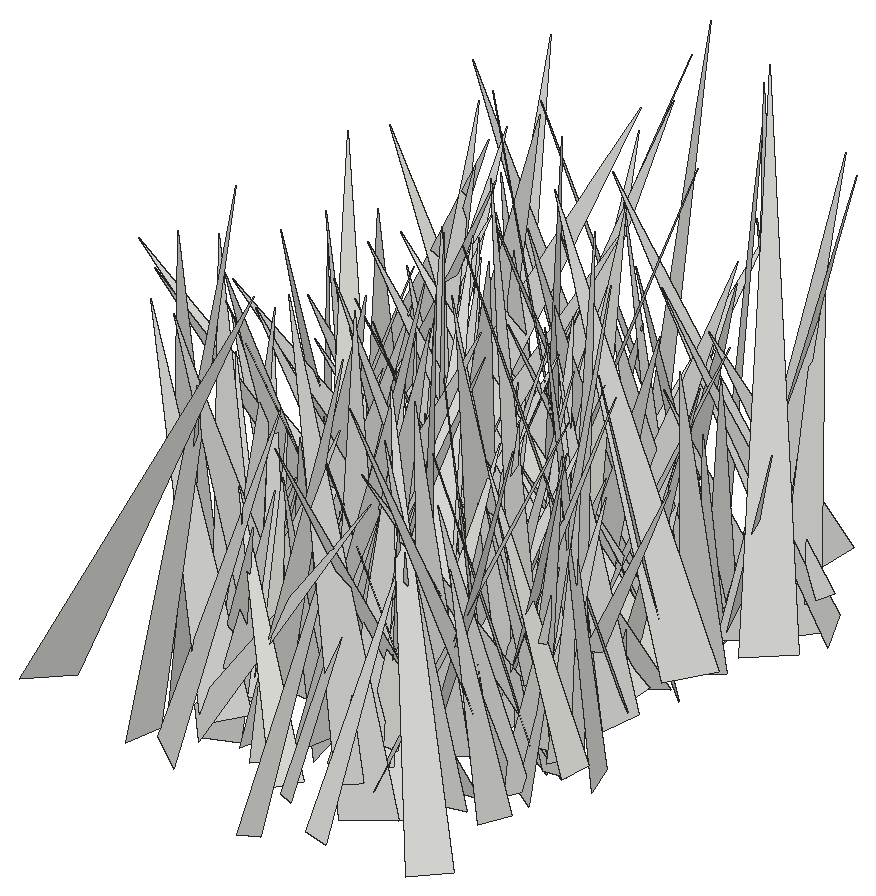
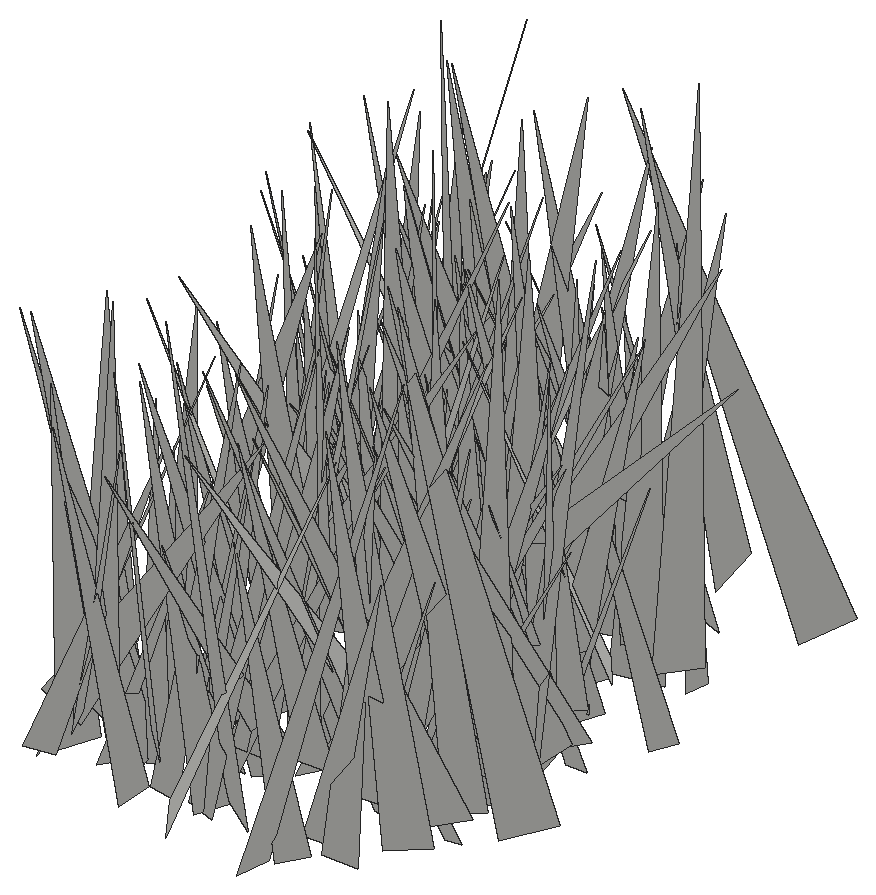
# SketchUp Ruby script. Lengths in inches.
U = 1.inch
M = Sketchup.active_model
def pt(a) = Geom::Point3d.new(a.map { |v| v * U })
def face(e, loops, mat)
  f = e.add_face(loops[0].map { |a| pt(a) })
  loops[1..].each { |l| e.add_face(l.map { |a| pt(a) }).erase! }
  f.material = f.back_material = mat if mat
  f
end
# faces: each face lists its corners as indices into pts; further lists are holes
def faces(e, pts, list, mat = nil) = list.each { |f| face(e, (f[0].is_a?(Array) ? f : [f]).map { |l| l.map { |i| pts[i] } }, mat) }
# xy, xz, yz: faces in a plane at the given z, y or x. An outline is a flat list of corners, or four numbers for a rectangle; further outlines are holes
def ring(l) = l.size == 4 ? [[l[0], l[1]], [l[2], l[1]], [l[2], l[3]], [l[0], l[3]]] : l.each_slice(2).to_a
def flat(e, list, mat, &to3) = list.each { |f| face(e, (f[0].is_a?(Array) ? f : [f]).map { |l| ring(l).map { |u, v| to3.(u, v) } }, mat) }
def xy(e, z, list, mat = nil) = flat(e, list, mat) { |x, y| [x, y, z] }
def xz(e, y, list, mat = nil) = flat(e, list, mat) { |x, z| [x, y, z] }
def yz(e, x, list, mat = nil) = flat(e, list, mat) { |y, z| [x, y, z] }
def lines(e, pts, list) = list.each { |a, b| e.add_line(pt(pts[a]), pt(pts[b])) }
# prism: a flat outline (further loops are holes) pulled along v
def prism(e, loops, v, mat = nil)
  f = face(e, loops, mat); d = Geom::Vector3d.new(v.map { |x| x * U })
  f.pushpull(f.normal.samedirection?(d) ? d.length : -d.length)
end
def box(e, o, s, mat = nil) = prism(e, [[o, [o[0] + s[0], o[1], o[2]], [o[0] + s[0], o[1] + s[1], o[2]], [o[0], o[1] + s[1], o[2]]]], [0, 0, s[2]], mat)
def at(x, y, z, deg = 0) = Geom::Transformation.translation(pt([x, y, z])) * Geom::Transformation.rotation(ORIGIN, Z_AXIS, deg.degrees)
def axes(o, x, y, z) = Geom::Transformation.new([*x, 0, *y, 0, *z, 0, *pt(o).to_a, 1])
def part(name) = M.definitions.add(name)
# library, detail: a bought-in or finely detailed component or shape, given as its bounding box
def library(name, o, s) = part(name).tap { |d| box(d.entities, o, s) }
def detail(e, o, s) = box(e.add_group.entities, o, s)
def put(e, d, t, mat = nil) = e.add_instance(d, t).tap { |i| i.material = mat if mat }
def group(e, t, mat = nil) = e.add_group.tap { |g| g.transformation = t; g.material = mat if mat }.entities
root = M.entities
c1 = part("fur_instance\#9")
p = [[0.8125,0,1.79],[0.67,-0.02,1.48],[0,-0.11,0],[0,0.11,0]]
faces(c1.entities,p,[[0,1,2,3]])
put(root,c1,axes([85.35,140.59,-27.1],[4.73655,-6.32836,0.37656],[-6.13582,-4.45802,2.25891],[1.59428,1.644,7.57499]))
put(root,c1,axes([88.57,135.68,-28.22],[5.38301,1.51294,2.42188],[1.75431,-5.82988,-0.25732],[-2.2532,-0.92457,5.58566]))
put(root,c1,axes([87.83,135.42,-28.22],[1.17442,4.10835,0.87727],[4.16659,-1.02282,-0.78793],[0.5364,-1.0501,4.19964]))
put(root,c1,axes([87.94,137.81,-28.22],[-2.59583,-7.17613,0.91864],[-6.91744,2.74775,1.9178],[2.11891,0.17907,7.38629]))
put(root,c1,axes([86.7,132.99,-28.22],[1.43751,-4.12245,0.23292],[-3.7226,-1.18725,1.96162],[1.78636,0.84328,3.90039]))
put(root,c1,axes([89.07,134.85,-28.22],[-3.37323,-1.69913,0.74168],[-1.13548,3.11072,1.96213],[1.46554,-1.50074,3.22735]))
put(root,c1,axes([90.43,138.84,-28.22],[-4.09373,-0.36711,0.23804],[-0.24891,3.79616,1.57392],[0.35983,-1.55061,3.79686]))
put(root,c1,axes([87.81,130.97,-27.1],[7.83218,-2.47016,1.5817],[-2.12062,-7.88445,-1.81244],[-2.02643,-1.29626,8.00998]))
put(root,c1,axes([89.42,141.9,-27.1],[-0.62472,6.74476,1.37593],[6.88336,0.62526,0.06028],[0.06565,-1.37569,6.77336]))
put(root,c1,axes([89.96,133.18,-27.1],[3.58153,-3.37168,2.12142],[-3.21603,-4.13077,-1.13573],[-2.3507,0.51427,4.78599]))
put(root,c1,axes([88.28,138.42,-28.22],[-2.09917,6.50868,2.06271],[6.47308,2.58358,-1.56477],[2.17184,-1.40938,6.65739]))
put(root,c1,axes([87.49,136.08,-27.1],[-0.99691,5.86129,1.26655],[5.41282,1.43213,-2.36709],[2.58075,-0.73958,5.45394]))
put(root,c1,axes([88.03,129.87,-28.22],[6.10646,0.88523,1.50787],[1.27518,-6.00248,-1.64024],[-1.19633,-1.87958,5.94829]))
put(root,c1,axes([89.45,139.24,-27.1],[5.03177,-2.92165,1.14225],[-2.20313,-4.82824,-2.64459],[-2.23316,-1.81978,5.18275]))
put(root,c1,axes([90.74,142.98,-28.22],[-2.03282,4.17049,1.29504],[4.34211,1.77825,1.08919],[-0.46493,-1.62705,4.50988]))
put(root,c1,axes([89.64,130.5,-28.22],[1.68119,-6.78383,2.85706],[-7.30642,-1.89388,-0.19753],[-0.89411,2.72073,6.98625]))
put(root,c1,axes([87.41,140.8,-27.1],[0.83878,-6.84447,1.51714],[-6.71971,-0.34936,2.13903],[1.99848,1.69801,6.55552]))
put(root,c1,axes([87.35,143.38,-27.1],[2.07111,-6.85146,1.31632],[-6.80663,-1.68294,1.94991],[1.53132,1.78604,6.88693]))
put(root,c1,axes([88.15,138.78,-27.1],[6.15158,-3.29467,0.71793],[-3.15743,-6.15236,-1.17953],[-1.18361,-0.7112,6.87789]))
put(root,c1,axes([86,126.67,-27.1],[7.56022,-3.29271,0.03526],[-3.23696,-7.41517,1.59297],[0.60437,1.47429,8.09082]))
put(root,c1,axes([91.37,138.15,-27.1],[-6.30471,-1.37126,0.42808],[-1.05468,5.72683,2.8114],[0.97532,-2.67133,5.80738]))
put(root,c1,axes([92.08,134.87,-27.1],[-0.45254,-7.13046,0.09555],[-6.72101,0.39447,-2.39372],[-2.38342,0.24148,6.7319]))
put(root,c1,axes([89.65,143.53,-28.22],[-0.39451,-5.89979,1.57703],[-6.09619,0.47415,0.24879],[0.36204,1.55494,5.90773]))
put(root,c1,axes([95.27,134.29,-28.22],[-5.86481,5.71927,0.12396],[4.62698,4.63811,4.91939],[-3.36399,-3.59156,6.55024]))
put(root,c1,axes([87.5,136.92,-27.1],[6.84085,-1.05323,0.60817],[-1.14548,-6.7472,1.19982],[-0.40871,1.28156,6.81667]))
put(root,c1,axes([91.27,145.3,-28.22],[-7.48109,-1.28394,1.71532],[-0.94889,7.57103,1.5286],[1.92105,-1.26035,7.43496]))
put(root,c1,axes([91.82,138.87,-27.1],[-4.16837,-0.36819,0.02902],[-0.35612,3.91965,-1.4217],[-0.09791,1.41863,3.93569]))
put(root,c1,axes([91.16,129.34,-27.1],[-3.95377,2.90545,0.68572],[2.92437,3.99824,-0.07937],[0.59996,-0.34142,4.90588]))
put(root,c1,axes([91.32,127.81,-27.1],[-4.7653,3.97573,1.88545],[4.327,4.73874,0.94381],[0.79899,-1.95123,6.13381]))
put(root,c1,axes([87.36,141.5,-27.1],[0.42432,7.03314,2.02201],[6.63788,0.48281,-3.07232],[3.08094,-2.00885,6.34082]))
put(root,c1,axes([90.99,139.2,-28.22],[-5.12264,0.34016,1.65759],[0.60899,5.30124,0.79415],[1.57874,-0.94118,5.07212]))
put(root,c1,axes([90.08,125.72,-27.1],[-7.4216,0.05563,3.73189],[-0.80703,8.0859,-1.72548],[3.64401,1.90407,7.21845]))
put(root,c1,axes([92.2,133,-27.1],[-6.19983,-0.76734,1.02255],[-1.02443,6.01091,-1.70052],[0.76483,1.83095,6.01123]))
put(root,c1,axes([89.79,130.11,-27.1],[5.47744,-1.647,1.93505],[-1.81976,-5.75174,0.25556],[-1.77356,0.81501,5.71398]))
put(root,c1,axes([89.24,132.125,-27.1],[4.55508,3.875,0.43107],[3.83788,-4.57312,0.55448],[-0.68713,0.14532,5.95457]))
put(root,c1,axes([91.71,132.8125,-27.1],[-3.76745,6.43232,1.47995],[6.58457,3.78058,0.33053],[0.45645,-1.44608,7.44709]))
put(root,c1,axes([91.01,130.72,-27.1],[4.14575,-5.15062,1.64406],[-4.88287,-4.45639,-1.64839],[-2.32151,0.17524,6.40304]))
put(root,c1,axes([93.28,139.89,-28.22],[-7.37091,1.53228,0.84327],[1.65266,7.29739,1.18581],[0.57246,-1.33774,7.43452]))
put(root,c1,axes([87.89,140.73,-28.22],[3.46284,5.45761,0.55951],[5.19477,-3.049,-2.40992],[1.76435,-1.73432,5.99742]))
put(root,c1,axes([90.61,133.84,-27.1],[1.9178,-7.47283,0.23219],[-7.45531,-1.92947,-0.52008],[-0.56157,0.09505,7.69744]))
put(root,c1,axes([93.1875,137.77,-28.22],[0.83306,-5.07313,1.39633],[-4.3947,-1.44829,-2.63999],[-2.89363,0.73905,4.41148]))
put(root,c1,axes([89.93,135.65,-28.22],[3.62066,0.28745,0.41277],[0.34104,-3.60783,-0.479],[-0.36973,-0.51296,3.60033]))
put(root,c1,axes([91.59,135.02,-27.1],[-6.63675,3.07759,1.929],[2.57186,6.8191,-2.03087],[2.56478,1.12578,7.02806]))
put(root,c1,axes([88.92,134.77,-27.1],[3.49272,-6.19271,0.17705],[-6.11252,-3.41157,1.25629],[1.00898,0.76914,6.99789]))
put(root,c1,axes([90.82,138.34,-28.22],[6.66219,5.05954,0.23915],[4.47229,-6.06129,3.64695],[-2.37798,2.77537,7.52884]))
put(root,c1,axes([90.65,129.59,-27.1],[2.6007,2.51832,0.88377],[2.64819,-2.58836,-0.41733],[-0.33183,-0.9193,3.59603]))
put(root,c1,axes([92.97,127.83,-27.1],[0.07199,5.81915,0.58708],[5.58747,-0.24194,1.7129],[-1.72841,-0.53974,5.5618]))
put(root,c1,axes([91.34,136.93,-28.22],[-0.57876,-6.04691,0.53315],[-6.05695,0.61084,0.35302],[0.40347,0.49606,6.06428]))
put(root,c1,axes([89.42,133.32,-28.22],[5.60342,-3.67276,1.04707],[-3.81273,-5.48708,1.15708],[-0.22057,1.54484,6.59914]))
put(root,c1,axes([89.85,133.125,-28.22],[0.06322,-6.05576,0.15688],[-5.74231,-0.00994,1.93043],[1.92942,0.16885,5.74018]))
put(root,c1,axes([89.73,129.66,-28.22],[0.93957,-4.99379,0.05949],[-4.70596,-0.86502,1.71172],[1.67197,0.37157,4.78443]))
put(root,c1,axes([89.64,129.64,-28.22],[2.95683,-4.48742,1.40063],[-4.613,-2.45121,1.88504],[0.90496,2.16707,5.03253]))
put(root,c1,axes([89.92,126.89,-28.22],[3.54049,4.95211,1.34575],[5.12044,-3.30078,-1.32493],[0.33991,-1.85767,5.94164]))
put(root,c1,axes([92.88,134.62,-27.1],[-6.34287,-0.8603,1.40577],[-0.30586,6.10717,2.3574],[1.61949,-2.21602,5.95103]))
put(root,c1,axes([90.05,140.86,-28.22],[3.15625,6.97995,0.87784],[7.00121,-3.02246,-1.14023],[0.68808,-1.26383,7.57506]))
put(root,c1,axes([90.68,128.4,-28.22],[3.21186,-3.52218,0.8528],[-3.62385,-3.13,0.72104],[-0.02677,1.11644,4.71189]))
put(root,c1,axes([94.8125,144.61,-28.22],[-5.86461,-3.9483,0.52207],[-3.9663,5.70596,-1.40208],[-0.36068,1.452,6.92942]))
put(root,c1,axes([91.9375,136.22,-27.1],[5.0258,-2.8928,2.35137],[-3.11716,-5.42578,-0.01254],[-2.04464,1.16127,5.79886]))
put(root,c1,axes([92.71,133.61,-27.1],[-4.05374,2.9207,0.15477],[2.65047,3.78022,-1.91631],[1.23673,1.47198,4.61422]))
put(root,c1,axes([92.18,141.37,-27.1],[0.04484,6.03011,0.93276],[6.10111,-0.02998,-0.09948],[0.09373,-0.93336,6.02946]))
put(root,c1,axes([90.71,144.26,-28.22],[3.52002,-2.83902,0.00242],[-2.82378,-3.50072,0.47096],[0.29379,0.3681,4.49764]))
put(root,c1,axes([91.37,134.81,-27.1],[3.19088,3.17646,1.19509],[3.39239,-3.03309,-0.99593],[-0.09903,-1.55252,4.39087]))
put(root,c1,axes([94.97,132.26,-28.22],[-4.92734,-5.46841,0.2776],[-5.45988,4.87887,-0.80338],[-0.41255,0.74316,7.31688]))
put(root,c1,axes([95.16,141.75,-28.22],[-3.66042,-4.84933,0.70173],[-4.78346,3.34689,-1.82316],[-1.06154,1.63996,5.79575]))
put(root,c1,axes([93.6,126.59,-27.1],[-4.4668,1.24969,0.75909],[0.98308,4.37301,-1.41442],[1.08236,1.18546,4.4174]))
put(root,c1,axes([91.31,135.1875,-28.22],[4.44559,-0.41699,0.42413],[-0.48383,-4.39553,0.74982],[-0.34594,0.78895,4.4017]))
put(root,c1,axes([91.24,133.01,-27.1],[1.22352,3.80068,0.33063],[3.61313,-1.04295,-1.38167],[1.22465,-0.72012,3.74608]))
put(root,c1,axes([94.63,136.87,-27.1],[-3.64802,-5.0358,0.07825],[-5.03596,3.64854,0.02575],[0.06676,0.04827,6.21825]))
put(root,c1,axes([94.9,126.02,-27.1],[-3.18645,2.79123,0.05753],[2.78151,3.16651,0.42911],[-0.23972,-0.36053,4.21429]))
put(root,c1,axes([94.1,133.01,-27.1],[2.37526,2.53476,1.46683],[2.25858,-2.78775,1.16004],[-1.86424,-0.14786,3.27432]))
put(root,c1,axes([93.22,129.76,-28.22],[4.6906,-0.13116,1.94102],[0.35682,-4.92253,-1.19491],[-1.91244,-1.24013,4.53774]))
put(root,c1,axes([95.32,133.8125,-28.22],[-2.38468,3.13652,0.12042],[3.02513,2.25628,1.13874],[-0.83714,-0.7813,3.77197]))
put(root,c1,axes([95.1,133.13,-27.1],[-5.93651,2.05948,0.4431],[1.83167,5.70073,-1.95618],[1.04056,1.71471,5.97135]))
put(root,c1,axes([92.86,139.95,-27.1],[6.58164,2.52237,2.667],[2.99732,-6.85363,-0.91486],[-2.11926,-1.85972,6.9888]))
put(root,c1,axes([93.49,143.21,-28.22],[4.31651,6.80061,2.35568],[7.01576,-4.58865,0.3914],[-1.60519,-1.76799,8.04533]))
put(root,c1,axes([95.23,138.75,-27.1],[-5.96506,-5.04673,2.13711],[-5.35643,6.03696,-0.69462],[1.15994,1.92465,7.7826]))
put(root,c1,axes([94.6,128.83,-27.1],[-4.83197,-1.5354,1.95575],[-2.0901,4.8234,-1.3772],[1.34681,1.9768,4.87942]))
put(root,c1,axes([92.46,134.65,-27.1],[0.05703,4.78722,0.58826],[4.57544,0.13244,-1.52137],[1.52606,-0.57598,4.5394]))
put(root,c1,axes([94.06,141.87,-27.1],[0.0355,-6.28923,0.69696],[-6.32457,-0.05728,-0.19472],[-0.19984,0.69551,6.28631]))
put(root,c1,axes([90.8,127.16,-27.1],[4.14208,3.82367,0.06036],[3.46383,-3.71363,-2.44781],[1.62049,-1.8356,5.07794]))
put(root,c1,axes([94.84,135.34,-27.1],[-4.07639,-4.57708,0.71562],[-4.52519,4.13816,0.69067],[0.99219,0.06853,6.09012]))
put(root,c1,axes([90.58,131.69,-28.22],[4.47531,-6.51665,1.20055],[-6.35255,-3.80729,3.0143],[1.88498,2.64087,7.30815]))
put(root,c1,axes([95.55,133.91,-27.1],[-6.52757,-2.25287,1.08541],[-2.07972,6.57544,1.14066],[1.38863,-0.74224,6.81054]))
put(root,c1,axes([94.42,143.6875,-28.22],[-2.90954,-6.16313,0.64564],[-6.10361,2.97343,0.8781],[1.07095,0.20243,6.75859]))
put(root,c1,axes([92.75,127.55,-27.1],[6.6153,-1.38256,1.33275],[-1.44359,-6.733,0.18083],[-1.26639,0.45296,6.75581]))
put(root,c1,axes([93.8125,130.55,-28.22],[3.60415,-6.43604,2.10161],[-6.7075,-3.71823,0.11619],[-0.92131,1.89247,7.37557]))
put(root,c1,axes([96.03,141.42,-27.1],[-5.27526,-0.92635,0.94955],[-1.13263,5.17215,-1.24665],[0.69057,1.40673,5.20887]))
put(root,c1,axes([98.01,138.26,-28.22],[-7.10232,2.48969,0.17848],[2.39972,6.66255,2.55443],[-0.68683,-2.46683,7.07929]))
put(root,c1,axes([95.06,134.58,-27.1],[-3.85021,0.78609,0.9669],[0.45373,3.80886,-1.28983],[1.16059,1.11875,3.71193]))
put(root,c1,axes([94.6,124.6875,-28.22],[-4.41851,1.16155,1.66424],[0.34777,4.36157,-2.12081],[1.99949,1.8082,4.04655]))
put(root,c1,axes([96.78,136.46,-27.1],[-7.42366,-0.80204,0.92134],[-0.52005,7.2098,2.08597],[1.1053,-1.9946,7.16957]))
put(root,c1,axes([95.62,130.31,-27.1],[-5.53054,0.45224,1.5037],[0.10523,5.59989,-1.29715],[1.5667,1.22031,5.39525]))
put(root,c1,axes([93.52,141.3125,-27.1],[-0.37436,5.47936,0.25355],[5.20879,0.43477,-1.70506],[1.71934,-0.12411,5.22075]))
put(root,c1,axes([92.49,136.95,-27.1],[2.66865,-7.95792,0.14871],[-7.80747,-2.5868,1.68053],[1.54726,0.67254,8.22351]))
put(root,c1,axes([94.28,132.76,-28.22],[3.35621,4.76804,0.53975],[4.75729,-3.3924,0.38655],[-0.62744,-0.21695,5.81798]))
put(root,c1,axes([95.13,132.32,-28.22],[4.5767,5.68819,3.18986],[6.17982,-5.02762,0.09872],[-2.08339,-2.41752,7.30013]))
put(root,c1,axes([95.61,140.58,-27.1],[-4.40501,-3.46188,0.56585],[-3.18391,4.32713,1.68747],[1.47225,-1.00011,5.34239]))
put(root,c1,axes([94.7,129.08,-28.22],[2.64907,4.14771,0.84835],[4.17625,-2.72433,0.27885],[-0.69438,-0.56151,4.91358]))
put(root,c1,axes([95.93,133.55,-27.1],[-3.80527,0.70423,0.62745],[0.3357,3.44844,-1.83447],[0.88144,1.72686,3.40746]))
put(root,c1,axes([94.76,133.82,-28.22],[3.48904,-1.79502,0.75996],[-1.60226,-3.52839,-0.97792],[-1.11014,-0.54905,3.7999]))
put(root,c1,axes([96.625,127.42,-28.22],[1.79805,-6.87497,3.712],[-7.43664,-2.674,-1.35027],[-2.39594,3.14033,6.97674]))
put(root,c1,axes([93.42,129.47,-27.1],[6.3266,0.04535,0.7535],[-0.10627,-6.24313,1.26797],[-0.74735,1.27161,6.1984]))
put(root,c1,axes([96.91,132.16,-28.22],[-4.58169,-0.00231,0.33908],[-0.10273,4.38765,-1.35823],[0.32316,1.36211,4.37574]))
put(root,c1,axes([95.07,133.85,-28.22],[0.28978,-3.77503,0.68612],[-3.83038,-0.24462,0.27184],[0.22308,0.70349,3.77636]))
put(root,c1,axes([95.32,125.41,-27.1],[3.44077,4.42208,0.21812],[4.18127,-3.33634,1.68138],[-1.45578,0.8691,5.34478]))
put(root,c1,axes([95.22,142.41,-27.1],[3.85472,-3.45884,0.89823],[-3.26491,-3.94586,-1.18314],[-1.45282,-0.30973,5.04209]))
put(root,c1,axes([95.17,141.24,-28.22],[0.89706,4.01856,0.51185],[4.05094,-0.89322,-0.08685],[-0.02607,-0.51851,4.11655]))
put(root,c1,axes([94.0625,128.22,-27.1],[7.6269,-0.50277,1.8471],[-0.68475,-7.80192,0.70374],[-1.78765,0.84341,7.61099]))
put(root,c1,axes([93.47,130.7,-27.1],[6.15872,-4.73604,0.69713],[-4.78091,-6.14284,0.50431],[-0.2428,0.82545,7.75278]))
put(root,c1,axes([97.04,128.87,-27.1],[-6.53703,2.92768,0.70077],[2.53956,6.26275,-2.47462],[1.61648,2.00045,6.72163]))
put(root,c1,axes([95.36,127.48,-27.1],[2.13777,3.57515,0.4757],[3.58502,-2.16686,0.17428],[-0.39447,-0.3179,4.1619]))
put(root,c1,axes([96.4,127.29,-27.1],[-5.56085,2.56326,1.5764],[2.25423,5.74256,-1.38556],[1.99343,0.65656,5.96435]))
put(root,c1,axes([95.77,143.58,-28.22],[-1.823,-5.96341,0.88128],[-5.94354,1.93183,0.77754],[1.00658,0.60664,6.18716]))
put(root,c1,axes([94.72,138.08,-28.22],[-2.73382,6.12597,3.74599],[6.6709,3.64992,-1.10045],[2.6569,-2.86083,6.61742]))
put(root,c1,axes([94.32,137.75,-28.22],[1.69765,-3.69471,0.41656],[-3.54176,-1.46758,1.41724],[1.13153,0.9496,3.81108]))
put(root,c1,axes([97.75,130.15,-28.22],[-1.10699,-6.38687,0.31821],[-6.26084,1.01671,-1.37367],[-1.30201,0.54128,6.33487]))
put(root,c1,axes([94.09,140.98,-28.22],[1.25839,-5.65908,2.69216],[-6.0262,-0.33916,2.10388],[1.71982,2.95233,5.40207]))
put(root,c1,axes([99.77,143.11,-27.1],[-2.20634,6.02099,1.75888],[5.48729,0.94934,3.63349],[-3.03901,-2.65713,5.28374]))
put(root,c1,axes([94.21,143.42,-28.22],[6.03259,-1.06555,0.38284],[-1.02373,-6.01977,-0.62323],[-0.48366,-0.54868,6.09418]))
put(root,c1,axes([97.31,127.98,-28.22],[-4.43994,6.98412,0.3729],[6.94517,4.45476,-0.74146],[0.82561,0.08476,8.24265]))
put(root,c1,axes([96.39,143.17,-27.1],[4.10758,4.73433,2.04961],[4.7509,-4.49256,0.85604],[-2.01089,-0.9434,6.20913]))
put(root,c1,axes([98.68,128.37,-27.1],[-3.99392,-3.16377,0.39905],[-3.06383,3.62986,-1.88605],[-0.88412,1.71311,4.73326]))
put(root,c1,axes([97.92,130.99,-28.22],[-2.14589,-4.13922,0.79032],[-4.13009,1.88974,-1.31675],[-0.83673,1.28775,4.4726]))
put(root,c1,axes([96.27,133.02,-28.22],[3.67967,2.76321,1.03507],[2.46473,-3.78797,1.35021],[-1.62229,0.51247,4.39911]))
put(root,c1,axes([95.47,134.33,-28.22],[0.23103,-4.99246,1.62863],[-5.17408,0.0623,0.92493],[0.89778,1.64376,4.91147]))
put(root,c1,axes([94.96,135.48,-28.22],[6.31463,-5.10403,0.36931],[-4.97216,-6.25818,-1.47472],[-1.21044,-0.91981,7.98441]))
put(root,c1,axes([96.125,125.74,-28.22],[1.13394,4.06883,0.24777],[4.07369,-1.14042,0.08414],[-0.14769,-0.216,4.22305]))
put(root,c1,axes([95.79,133.27,-27.1],[6.81061,4.1437,0.72104],[3.52808,-6.3754,3.31382],[-2.28972,2.50169,7.25074]))
put(root,c1,axes([97.68,132.78,-27.1],[-6.3571,-0.05635,1.63328],[-0.03082,6.56286,0.10646],[1.63396,-0.09544,6.35645]))
put(root,c1,axes([94.75,139.37,-27.1],[4.6953,-3.04636,0.27903],[-3.0591,-4.67738,0.40996],[-0.01004,0.49581,5.58194]))
put(root,c1,axes([95.52,130.34,-28.22],[5.31663,-1.02418,0.76649],[-0.77202,-5.18142,-1.56841],[-1.02002,-1.41668,5.18224]))
put(root,c1,axes([96.62,135.16,-27.1],[-2.20726,4.7722,2.01563],[5.04733,2.47451,-0.33147],[1.16667,-1.67676,5.24748]))
put(root,c1,axes([96.58,129.2,-27.1],[-2.91269,3.59929,0.76549],[3.33369,2.99435,-1.39463],[1.55801,0.3218,4.41516]))
put(root,c1,axes([98.8125,131.9,-27.1],[1.70019,7.5386,2.42367],[7.33263,-2.43467,2.42902],[-2.9895,-1.68439,7.33628]))
put(root,c1,axes([96.32,128.23,-27.1],[-1.6675,3.7386,1.84502],[3.94069,2.06209,-0.61692],[1.36097,-1.39013,4.04687]))
put(root,c1,axes([96.51,130.75,-27.1],[-3.43381,3.18637,0.41007],[2.54254,3.06224,-2.50406],[1.96382,1.60682,3.959]))
put(root,c1,axes([98.24,138.11,-28.22],[-0.29394,-4.28793,0.2812],[-4.0742,0.18848,-1.38464],[-1.36614,0.36048,4.06885]))
put(root,c1,axes([97.5625,135.52,-28.22],[-3.35833,-3.2337,1.73378],[-3.57177,3.41915,-0.54142],[0.83981,1.61055,4.63056]))
put(root,c1,axes([98.0625,139.54,-28.22],[-3.41179,-1.77285,0.16017],[-1.67154,3.30984,1.02951],[0.61205,-0.84317,3.70451]))
put(root,c1,axes([96.01,130.08,-28.22],[-0.53016,-5.209,0.61736],[-4.97847,0.69512,1.58982],[1.65216,0.4231,4.98871]))
put(root,c1,axes([96.35,130.04,-27.1],[7.03768,2.72348,2.80411],[3.28727,-7.24831,-1.21043],[-2.11523,-2.20318,7.44856]))
put(root,c1,axes([96.23,133,-27.1],[3.37327,4.28522,1.21914],[4.44713,-3.33099,-0.5966],[-0.2692,-1.33033,5.4209]))
put(root,c1,axes([97.23,136.4,-28.22],[2.55514,-3.36467,0.69917],[-3.31318,-2.64324,-0.61213],[-0.91251,0.1757,4.18031]))
put(root,c1,axes([98.09,143.23,-28.22],[-4.22859,-0.79072,0.99748],[-0.41595,4.12901,1.5098],[1.20299,-1.35177,4.02824]))
put(root,c1,axes([97.37,141.81,-28.22],[0.8315,-3.67241,0.7269],[-3.73531,-0.86356,-0.09004],[-0.24991,0.6885,3.76429]))
put(root,c1,axes([96.34,144.21,-28.22],[5.61379,-0.0924,1.25595],[-0.17391,-5.73971,0.3551],[-1.24727,0.38445,5.60331]))
put(root,c1,axes([99.76,137.63,-27.1],[-4.16416,5.80884,2.0419],[6.1268,3.66414,2.07088],[-0.6118,-2.84317,6.84063]))
put(root,c1,axes([98.45,142.89,-27.1],[1.87849,6.8023,2.53671],[7.02619,-2.36292,1.13321],[-1.82724,-2.09291,6.96533]))
put(root,c1,axes([98.64,135.98,-28.22],[-5.40914,1.11965,1.3835],[1.23539,5.5484,0.3398],[1.28121,-0.62292,5.51334]))
put(root,c1,axes([98.96,143.34,-27.1],[-4.99068,-1.45127,1.21381],[-1.71677,4.91279,-1.18474],[0.79513,1.49823,5.06058]))
put(root,c1,axes([97.27,129.89,-27.1],[3.86717,-5.0611,1.49434],[-5.13106,-4.03908,-0.40116],[-1.23289,0.93486,6.35679]))
put(root,c1,axes([98.72,130.25,-27.1],[3.89411,3.28531,3.07479],[3.51498,-4.75969,0.63397],[-2.80935,-1.40135,5.05524]))
put(root,c1,axes([98.88,135.65,-27.1],[-4.98525,-6.36904,1.05647],[-6.36247,5.07321,0.56124],[1.09531,0.48105,8.06861]))
put(root,c1,axes([98.55,133.53,-28.22],[-5.64756,-4.03637,0.24701],[-3.60758,5.22048,2.82493],[1.82721,-2.16853,6.3409]))
put(root,c1,axes([98.33,134.1875,-28.22],[3.17531,6.56755,2.54139],[6.79761,-3.58673,0.77578],[-1.83954,-1.91744,7.25351]))
put(root,c1,axes([98.72,145.36,-27.1],[3.46257,-3.0651,1.27719],[-2.41097,-3.5895,-2.07802],[-2.28326,-0.85797,4.13111]))
put(root,c1,axes([97.21,141.75,-28.22],[-0.07367,-4.26522,0.50041],[-4.16979,0.19077,1.01214],[1.02732,0.46845,4.14405]))
put(root,c1,axes([97.04,142.4,-28.22],[0.2797,-5.08952,0.70223],[-5.01624,-0.11848,1.13926],[1.11073,0.74654,4.96825]))
put(root,c1,axes([99.02,132.6,-28.22],[-0.77658,-4.10323,1.17838],[-4.23531,0.59015,-0.73621],[-0.53592,1.28194,4.11067]))
put(root,c1,axes([99.17,127.79,-27.1],[-0.52973,-5.32119,2.08202],[-5.65742,0.19488,-0.94137],[-0.8022,2.1395,5.26399]))
put(root,c1,axes([98.46,132.16,-27.1],[-3.60567,-4.25836,0.82426],[-4.10665,3.69659,1.13335],[1.39586,-0.12438,5.46351]))
put(root,c1,axes([95.91,137.86,-27.1],[5.05169,2.87341,0.23488],[2.86098,-4.93803,-1.1233],[0.35552,-1.09113,5.70213]))
put(root,c1,axes([97.1875,137.76,-28.22],[5.08569,0.11573,0.95874],[0.07501,-5.17107,0.22632],[-0.96278,0.20845,5.08197]))
put(root,c1,axes([99.97,143.66,-28.22],[-5.70608,-2.81682,0.48614],[-2.67601,5.6456,1.30244],[1.0049,-0.96065,6.22877]))
put(root,c1,axes([98.44,138.5,-28.22],[-3.34858,-4.98605,1.16696],[-4.83329,3.53804,1.24784],[1.69169,0.23891,5.87509]))
put(root,c1,axes([98.75,130.94,-28.22],[-3.71631,2.59474,2.95715],[3.6126,3.86147,1.15179],[1.55775,-2.76492,4.38373]))
put(root,c1,axes([101.08,124.54,-27.1],[-1.83761,6.5724,0.07775],[6.30696,1.74042,1.94227],[-1.85059,-0.59481,6.54223]))
put(root,c1,axes([100.7,139.89,-27.1],[-7.32021,3.8589,0.48336],[3.73123,7.2592,-1.44642],[1.09666,1.05977,8.14767]))
put(root,c1,axes([98.95,130.55,-27.1],[-6.12859,-4.53414,1.24355],[-3.97845,6.08997,2.59781],[2.50535,-1.42065,7.16724]))
put(root,c1,axes([97.29,142.45,-28.22],[6.99973,1.86447,1.44835],[1.77883,-7.14461,0.6004],[-1.55233,0.22015,7.21886]))
put(root,c1,axes([97.16,135.23,-28.22],[4.11337,-1.35782,0.42666],[-1.42017,-4.00175,0.95638],[-0.09392,1.04301,4.22479]))
put(root,c1,axes([98.31,133.125,-27.1],[-2.24113,2.46388,1.48853],[2.36542,2.65133,-0.82724],[1.6405,-0.45695,3.22631]))
put(root,c1,axes([98.32,141.7,-28.22],[6.53232,-2.04401,3.08815],[-2.89411,-6.72439,1.67109],[-2.31057,2.64395,6.63752]))
put(root,c1,axes([96.9375,132.0625,-27.1],[4.58071,3.98416,0.78034],[4.05613,-4.44078,-1.1369],[0.17387,-1.36793,5.96354]))
put(root,c1,axes([96.59,127.875,-27.1],[5.74165,3.30721,0.02247],[3.30582,-5.73764,-0.2359],[0.09829,-0.21562,6.62182]))
put(root,c1,axes([100.63,131.47,-27.1],[-4.67838,0.58429,0.4377],[0.60816,4.68963,0.24018],[0.40387,-0.29353,4.7086]))
put(root,c1,axes([96.875,129.87,-27.1],[6.48852,0.93317,0.66882],[1.0636,-6.33108,-1.48501],[-0.43231,-1.57025,6.38486]))
put(root,c1,axes([99.04,131.11,-28.22],[4.31579,6.0344,1.65644],[5.97789,-4.5707,1.07586],[-1.85004,-0.69181,7.34048]))
put(root,c1,axes([98.53,131.32,-28.22],[3.38987,-1.12165,1.00676],[-1.27426,-3.45624,0.43994],[-0.80492,0.7478,3.54341]))
put(root,c1,axes([100.2,133.07,-28.22],[5.38161,2.47127,3.67462],[2.66712,-6.4254,0.41515],[-3.53503,-1.08568,5.90733]))
put(root,c1,axes([99.38,142.85,-28.22],[4.97353,-2.18793,2.98402],[-2.79783,-5.49524,0.634],[-2.42149,1.85546,5.39639]))
put(root,c1,axes([99.33,129.58,-28.22],[3.16597,-2.82128,1.36449],[-2.73379,-3.43456,-0.75836],[-1.53229,0.2984,4.17228]))
put(root,c1,axes([98.6875,139.54,-28.22],[3.24454,-4.71501,1.03025],[-4.7617,-3.32972,-0.24278],[-0.78672,0.70811,5.71834]))
put(root,c1,axes([97.86,141.85,-28.22],[4.14097,0.37336,0.37849],[0.46882,-3.96604,-1.21698],[-0.25072,-1.24957,3.97567]))
put(root,c1,axes([96.75,133.51,-27.1],[6.70588,0.95076,0.50826],[1.07552,-6.12086,-2.74035],[-0.07444,-2.78609,6.19381]))
put(root,c1,axes([99.87,131.6875,-27.1],[-4.04138,0.55951,1.25439],[0.25517,4.13619,-1.02282],[1.34961,0.89343,3.94964]))
put(root,c1,axes([98.02,132.95,-28.22],[-1.36067,-5.7583,1.83351],[-5.61411,1.9,1.80082],[2.23642,1.26617,5.63617]))
